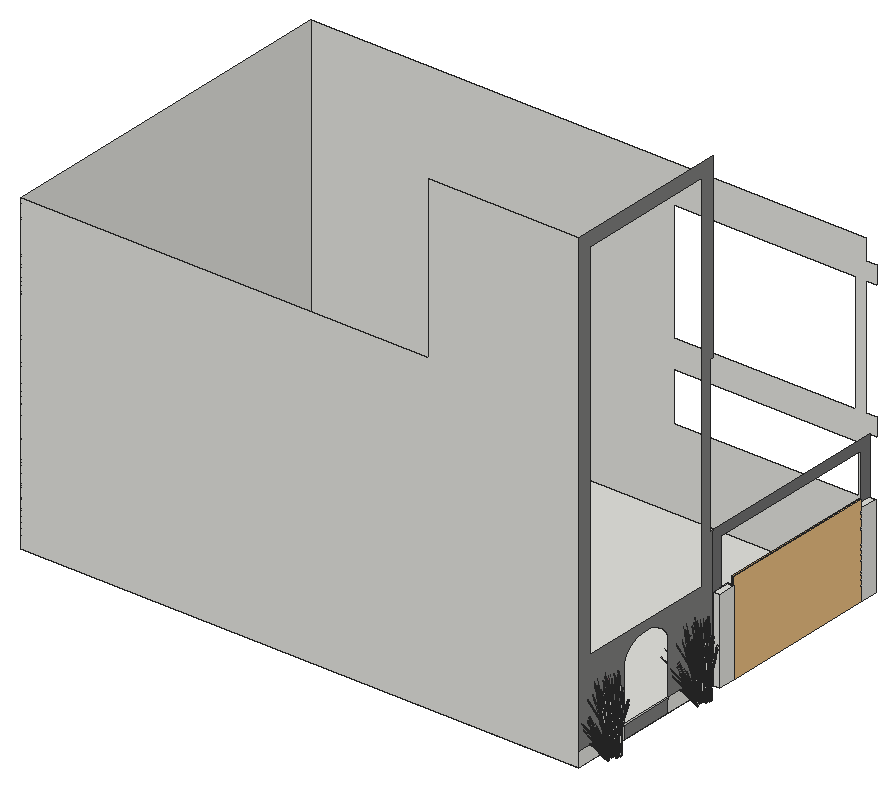
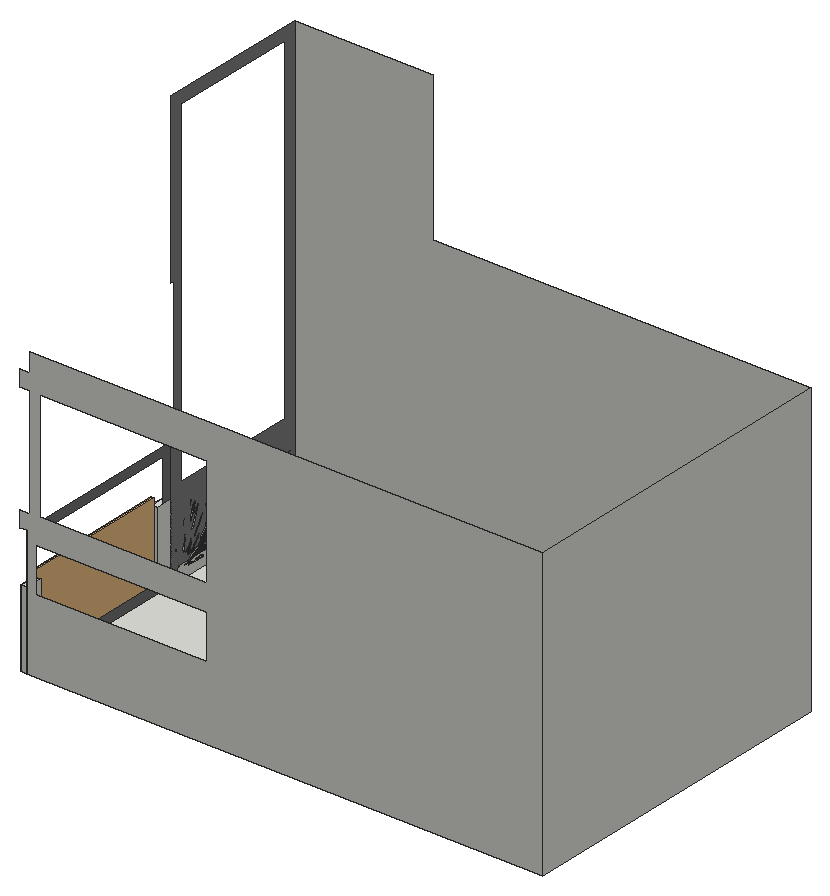
# SketchUp Ruby script. Lengths in inches.
U = 1.inch
M = Sketchup.active_model
def pt(a) = Geom::Point3d.new(a.map { |v| v * U })
def face(e, loops, mat)
  f = e.add_face(loops[0].map { |a| pt(a) })
  loops[1..].each { |l| e.add_face(l.map { |a| pt(a) }).erase! }
  f.material = f.back_material = mat if mat
  f
end
# faces: each face lists its corners as indices into pts; further lists are holes
def faces(e, pts, list, mat = nil) = list.each { |f| face(e, (f[0].is_a?(Array) ? f : [f]).map { |l| l.map { |i| pts[i] } }, mat) }
# xy, xz, yz: faces in a plane at the given z, y or x. An outline is a flat list of corners, or four numbers for a rectangle; further outlines are holes
def ring(l) = l.size == 4 ? [[l[0], l[1]], [l[2], l[1]], [l[2], l[3]], [l[0], l[3]]] : l.each_slice(2).to_a
def flat(e, list, mat, &to3) = list.each { |f| face(e, (f[0].is_a?(Array) ? f : [f]).map { |l| ring(l).map { |u, v| to3.(u, v) } }, mat) }
def xy(e, z, list, mat = nil) = flat(e, list, mat) { |x, y| [x, y, z] }
def xz(e, y, list, mat = nil) = flat(e, list, mat) { |x, z| [x, y, z] }
def yz(e, x, list, mat = nil) = flat(e, list, mat) { |y, z| [x, y, z] }
def lines(e, pts, list) = list.each { |a, b| e.add_line(pt(pts[a]), pt(pts[b])) }
# prism: a flat outline (further loops are holes) pulled along v
def prism(e, loops, v, mat = nil)
  f = face(e, loops, mat); d = Geom::Vector3d.new(v.map { |x| x * U })
  f.pushpull(f.normal.samedirection?(d) ? d.length : -d.length)
end
def box(e, o, s, mat = nil) = prism(e, [[o, [o[0] + s[0], o[1], o[2]], [o[0] + s[0], o[1] + s[1], o[2]], [o[0], o[1] + s[1], o[2]]]], [0, 0, s[2]], mat)
def at(x, y, z, deg = 0) = Geom::Transformation.translation(pt([x, y, z])) * Geom::Transformation.rotation(ORIGIN, Z_AXIS, deg.degrees)
def axes(o, x, y, z) = Geom::Transformation.new([*x, 0, *y, 0, *z, 0, *pt(o).to_a, 1])
def part(name) = M.definitions.add(name)
# library, detail: a bought-in or finely detailed component or shape, given as its bounding box
def library(name, o, s) = part(name).tap { |d| box(d.entities, o, s) }
def detail(e, o, s) = box(e.add_group.entities, o, s)
def put(e, d, t, mat = nil) = e.add_instance(d, t).tap { |i| i.material = mat if mat }
def group(e, t, mat = nil) = e.add_group.tap { |g| g.transformation = t; g.material = mat if mat }.entities
root = M.entities
M.materials.add("LightPink_Translucent").color = [144, 107, 117]
M.materials["LightPink_Translucent"].alpha = 0.75
M.materials.add("M05_Graphite_Haze").color = [114, 114, 114]
M.materials.add("ThomThom - Waistcoat2").color = [127, 127, 126]
c1 = part("blade")
p = [[2.15,0.21,22],[0,0.17,0],[0.09,0.45,0],[2.18,0.31,22],[2.29,0.31,22],[0.38,0.45,0],
  [2.48,0.24,33],[2.49,0.24,33],[2.48,0.22,33]]
faces(c1.entities,p,[[0,1,2,3],[4,5,2,3],[6,3,4,7],[8,0,3,6]])
c2 = part("seeds")
p = [[0.3,-0.1,1.38],[-0.01,-0.03,1.59],[-0.01,-0.03,0.03],[0.14,-0.07,-0.07],[0.29,-0.03,3],[0.15,0.01,3.11]]
faces(c2.entities,p,[[0,1,2,3],[1,0,4,5]],"LightPink_Translucent")
c3 = part("blade with seeds")
put(c3.entities,c1,at(0,0,0))
put(c3.entities,c2,axes([2.4,0.25,30.99],[1.5799,-0.05474,1.17369],[-0.12525,1.92788,0.29478],[-0.07173,-0.02425,1.56792]))
c4 = library("Modern+Gate+1",[0,0,0],[118.11,1.97,78.74])
box(root,[480,144,0],[6,15.46,72])
box(root,[480,295.78,0],[6,15.46,72])
xy(root,0,[[0,0,480,312]])
xz(root,0,[[0,0,480,0,480,408,351.33,408,351.33,270,0,270]])
xz(root,312,[[[0,0,0,270,477,270,477,252,486,252,486,237,312,237,312,135,468,135,468,237,477,237,477,135,486,135,486,120,480,120,480,0],[312,69,471,111]]])
yz(root,0,[[0,0,312,270]])
yz(root,480,[[0,0,48,0,48,11.26,96,11.26,96,12,0,12],[96,0,136.05,12]])
yz(root,480,[[[144,0,312,120],[153,9,303,111]]],"M05_Graphite_Haze")
yz(root,480,[[[136.05,0,144,0,144,120,141,120,141,252,144,252,144,408,0,408,0,12,48,12,48,60,50.74,64,54.14,67.47,58.1,70.28,62.48,72.35,67.17,73.62,72,74.05,76.83,73.62,81.52,72.35,85.9,70.28,89.86,67.47,93.26,64,96,60,96,12,136.05,12],[12,81.33,132,396]],[48,0,96,11.26]],"ThomThom - Waistcoat2")
put(root,c3,axes([486.59,117.58,3.875],[0.50831,-0.02346,1.71376],[-0.33721,1.01661,0.13857],[-0.72439,-0.06288,0.73262]))
put(root,c3,axes([486.59,21.58,3.875],[0.50831,-0.02346,1.71376],[-0.33721,1.01661,0.13857],[-0.72439,-0.06288,0.73262]))
put(root,c3,axes([486.8,119.375,3.875],[0.42521,-0.21906,1.71376],[0.35798,1.01226,0.13857],[-0.66754,0.22878,0.73262]))
put(root,c3,axes([486.8,23.375,3.875],[0.42521,-0.21906,1.71376],[0.35798,1.01226,0.13857],[-0.66754,0.22878,0.73262]))
put(root,c3,axes([485.48,121.1,2.59],[0.42589,0.08502,1.43002],[0.2745,0.86839,-0.30754],[-0.57851,0.16255,0.61141]))
put(root,c3,axes([485.48,25.1,2.59],[0.42589,0.08502,1.43002],[0.2745,0.86839,-0.30754],[-0.57851,0.16255,0.61141]))
put(root,c3,axes([489.25,118.32,3.34],[0.34834,-0.14982,1.77064],[0.12012,1.04605,0.13857],[-0.75452,0.1388,0.63284]))
put(root,c3,axes([489.25,22.32,3.34],[0.34834,-0.14982,1.77064],[0.12012,1.04605,0.13857],[-0.75452,0.1388,0.63284]))
put(root,c3,axes([488.11,116.64,4.98],[-1.22504,-0.02494,-0.71045],[0.08228,-1.05005,0.08574],[-0.51899,-0.11081,1.00501]))
put(root,c3,axes([488.11,20.64,4.98],[-1.22504,-0.02494,-0.71045],[0.08228,-1.05005,0.08574],[-0.51899,-0.11081,1.00501]))
put(root,c3,axes([487.125,116.9,2.59],[0.23927,0.28834,1.43002],[-0.55135,0.78376,-0.30754],[-0.56612,-0.18733,0.61141]))
put(root,c3,axes([487.125,20.9,2.59],[0.23927,0.28834,1.43002],[-0.55135,0.78376,-0.30754],[-0.56612,-0.18733,0.61141]))
put(root,c3,axes([486.14,118.46,4.53],[-1.01846,-0.28891,-0.35414],[0.29705,-0.84289,0.4572],[-0.41005,0.07729,0.87481]))
put(root,c3,axes([486.14,22.46,4.53],[-1.01846,-0.28891,-0.35414],[0.29705,-0.84289,0.4572],[-0.41005,0.07729,0.87481]))
put(root,c3,axes([487.55,115.95,3.875],[0.45521,0.17844,1.71376],[-0.94204,0.74856,0.13857],[-0.58713,-0.33769,0.73262]))
put(root,c3,axes([487.55,19.95,3.875],[0.45521,0.17844,1.71376],[-0.94204,0.74856,0.13857],[-0.58713,-0.33769,0.73262]))
put(root,c3,axes([486.84,118.89,4.68],[-0.332,0.94205,-0.51099],[-1.13828,-0.3229,-0.3958],[-0.45829,0.08638,0.97773]))
put(root,c3,axes([486.84,22.89,4.68],[-0.332,0.94205,-0.51099],[-1.13828,-0.3229,-0.3958],[-0.45829,0.08638,0.97773]))
put(root,c3,axes([487.7,116.85,4.68],[-0.88986,0.68603,-0.51099],[-0.77932,-0.72471,-0.3958],[-0.45212,-0.10438,0.97773]))
put(root,c3,axes([487.7,20.85,4.68],[-0.88986,0.68603,-0.51099],[-0.77932,-0.72471,-0.3958],[-0.45212,-0.10438,0.97773]))
put(root,c3,axes([486.27,118.83,1.49],[0.03108,0.16322,1.76342],[-0.62654,0.85237,-0.26939],[-0.44504,-0.04296,0.30037]))
put(root,c3,axes([486.27,22.83,1.49],[0.03108,0.16322,1.76342],[-0.62654,0.85237,-0.26939],[-0.44504,-0.04296,0.30037]))
put(root,c3,axes([484.59,122.92,2.77],[0.51072,-0.46938,1.1486],[0.20153,0.74307,0.84392],[-0.36908,0.13305,0.25299]))
put(root,c3,axes([484.59,26.92,2.77],[0.51072,-0.46938,1.1486],[0.20153,0.74307,0.84392],[-0.36908,0.13305,0.25299]))
put(root,c3,axes([487.375,116.21,4.53],[-0.69728,-0.64842,-0.35414],[0.79619,-0.61382,0.4572],[-0.40453,-0.09339,0.87481]))
put(root,c3,axes([487.375,20.21,4.53],[-0.69728,-0.64842,-0.35414],[0.79619,-0.61382,0.4572],[-0.40453,-0.09339,0.87481]))
put(root,c3,axes([488.36,120.06,3.875],[0.30609,-0.31822,1.71376],[0.77286,0.85893,0.13857],[-0.53009,0.39116,0.73262]))
put(root,c3,axes([488.36,24.06,3.875],[0.30609,-0.31822,1.71376],[0.77286,0.85893,0.13857],[-0.53009,0.39116,0.73262]))
put(root,c3,axes([486.52,120.89,4.53],[-1.06674,0.14801,-0.35414],[-0.28168,-0.84611,0.4572],[-0.30569,0.22726,0.87481]))
put(root,c3,axes([486.52,24.89,4.53],[-1.06674,0.14801,-0.35414],[-0.28168,-0.84611,0.4572],[-0.30569,0.22726,0.87481]))
put(root,c3,axes([485.93,123.4,1.49],[0.16438,0.10347,1.76342],[0.27873,0.95868,-0.26939],[-0.36432,0.20444,0.30037]))
put(root,c3,axes([485.93,27.4,1.49],[0.16438,0.10347,1.76342],[0.27873,0.95868,-0.26939],[-0.36432,0.20444,0.30037]))
put(root,c3,axes([485.7,117.76,2.77],[0.78239,-0.07411,1.1486],[-0.49629,0.65296,0.84392],[-0.38663,-0.09795,0.25299]))
put(root,c3,axes([485.7,21.76,2.77],[0.78239,-0.07411,1.1486],[-0.49629,0.65296,0.84392],[-0.38663,-0.09795,0.25299]))
put(root,c3,axes([488.13,120.84,3.875],[0.22818,-0.35597,1.71376],[0.95725,0.73667,0.13857],[-0.43183,0.45914,0.73262]))
put(root,c3,axes([488.13,24.84,3.875],[0.22818,-0.35597,1.71376],[0.95725,0.73667,0.13857],[-0.43183,0.45914,0.73262]))
put(root,c3,axes([487.4,120.99,4.68],[0.31482,0.94565,-0.51099],[-1.19224,0.16542,-0.3958],[-0.34166,0.254,0.97773]))
put(root,c3,axes([487.4,24.99,4.68],[0.31482,0.94565,-0.51099],[-1.19224,0.16542,-0.3958],[-0.34166,0.254,0.97773]))
put(root,c3,axes([490.37,120.31,2.06],[-1.27479,-0.1698,-0.62353],[0.26901,-1.04736,-0.16365],[-0.38043,-0.12691,1.37633]))
put(root,c3,axes([490.37,24.31,2.06],[-1.27479,-0.1698,-0.62353],[0.26901,-1.04736,-0.16365],[-0.38043,-0.12691,1.37633]))
put(root,c3,axes([490.24,115.4,4.98],[-1.04497,-0.50058,-0.71045],[0.74264,-0.8772,0.08574],[-0.3786,-0.29889,1.00501]))
put(root,c3,axes([490.24,19.4,4.98],[-1.04497,-0.50058,-0.71045],[0.74264,-0.8772,0.08574],[-0.3786,-0.29889,1.00501]))
put(root,c3,axes([489.75,115.43,4.68],[-1.20928,0.24619,-0.51099],[-0.21154,-0.93233,-0.3958],[-0.32481,-0.26718,0.97773]))
put(root,c3,axes([489.75,19.43,4.68],[-1.20928,0.24619,-0.51099],[-0.21154,-0.93233,-0.3958],[-0.32481,-0.26718,0.97773]))
put(root,c3,axes([488.7,122.29,2.02],[-1.14694,-0.51783,-0.49651],[0.68554,-0.92854,0],[-0.26122,-0.11794,1.57504]))
put(root,c3,axes([488.7,26.29,2.02],[-1.14694,-0.51783,-0.49651],[0.68554,-0.92854,0],[-0.26122,-0.11794,1.57504]))
put(root,c3,axes([488.19,114.58,1.49],[-0.11871,0.13643,1.76342],[-1.19964,0.29415,-0.26939],[-0.2898,-0.26759,0.30037]))
put(root,c3,axes([488.19,18.58,1.49],[-0.11871,0.13643,1.76342],[-1.19964,0.29415,-0.26939],[-0.2898,-0.26759,0.30037]))
put(root,c3,axes([489.39,122.92,2.375],[-0.7662,1.03778,0],[-1.28187,-0.57875,-0.51607],[-0.29196,-0.13181,1.63711]))
put(root,c3,axes([489.39,26.92,2.375],[-0.7662,1.03778,0],[-1.28187,-0.57875,-0.51607],[-0.29196,-0.13181,1.63711]))
put(root,c3,axes([488,124.42,2.59],[0.38672,-0.16338,1.43002],[0.95481,0.49262,-0.30754],[-0.28419,0.42626,0.61141]))
put(root,c3,axes([488,28.42,2.59],[0.38672,-0.16338,1.43002],[0.95481,0.49262,-0.30754],[-0.28419,0.42626,0.61141]))
put(root,c3,axes([487.45,115.1,2.13],[-0.35352,0.84566,-0.03893],[-1.08806,-0.26014,-0.17649],[-0.1652,-0.13832,0.58215]))
put(root,c3,axes([487.45,19.1,2.13],[-0.35352,0.84566,-0.03893],[-1.08806,-0.26014,-0.17649],[-0.1652,-0.13832,0.58215]))
put(root,c3,axes([489.07,114.04,2.59],[-0.07421,0.33879,1.43002],[-1.08488,0.28361,-0.30754],[-0.25359,-0.4379,0.61141]))
put(root,c3,axes([489.07,18.04,2.59],[-0.07421,0.33879,1.43002],[-1.08488,0.28361,-0.30754],[-0.25359,-0.4379,0.61141]))
put(root,c3,axes([489.43,114.92,3.875],[0.28013,0.33252,1.71376],[-1.29445,0.27994,0.13857],[-0.29256,-0.52202,0.73262]))
put(root,c3,axes([489.43,18.92,3.875],[0.28013,0.33252,1.71376],[-1.29445,0.27994,0.13857],[-0.29256,-0.52202,0.73262]))
put(root,c3,axes([491.8125,120.46,2.67],[-1.23732,0.68758,-0.29095],[-0.8228,-0.97154,-0.50002],[-0.30528,-0.09867,1.59708]))
put(root,c3,axes([491.8125,24.46,2.67],[-1.23732,0.68758,-0.29095],[-0.8228,-0.97154,-0.50002],[-0.30528,-0.09867,1.59708]))
put(root,c3,axes([489.88,114.74,4.53],[-0.18927,-0.83419,-0.35414],[1.08199,-0.22027,0.4572],[-0.29062,-0.23905,0.87481]))
put(root,c3,axes([489.88,18.74,4.53],[-0.18927,-0.83419,-0.35414],[1.08199,-0.22027,0.4572],[-0.29062,-0.23905,0.87481]))
put(root,c3,axes([486.86,118.96,2.375],[-1.53239,0,0],[0,-1.1575,-0.51607],[0,-0.26363,1.63711]))
put(root,c3,axes([486.86,22.96,2.375],[-1.53239,0,0],[0,-1.1575,-0.51607],[0,-0.26363,1.63711]))
put(root,c3,axes([489.01,121.9,2.03],[-0.28787,-0.90242,-0.30978],[1.14332,-0.25625,0.30978],[-0.23049,-0.10406,1.38974]))
put(root,c3,axes([489.01,25.9,2.03],[-0.28787,-0.90242,-0.30978],[1.14332,-0.25625,0.30978],[-0.23049,-0.10406,1.38974]))
put(root,c3,axes([488.39,122.85,4.53],[-0.82919,0.54528,-0.35414],[-0.78493,-0.62262,0.4572],[-0.11943,0.31634,0.87481]))
put(root,c3,axes([488.39,26.85,4.53],[-0.82919,0.54528,-0.35414],[-0.78493,-0.62262,0.4572],[-0.11943,0.31634,0.87481]))
put(root,c4,axes([486,159.46,0],[0,1.15423,0],[-1,0,0],[0,0,1]))
put(root,c3,axes([492.64,121.21,2.06],[-0.82544,0.77843,-0.62353],[-1.0254,-0.70586,-0.16365],[-0.33076,0.19418,1.37633]))
put(root,c3,axes([492.64,25.21,2.06],[-0.82544,0.77843,-0.62353],[-1.0254,-0.70586,-0.16365],[-0.33076,0.19418,1.37633]))
put(root,c3,axes([488.05,118.66,2.33],[-1.1399,0.87071,0.30756],[-1.1406,-0.86155,-0.36492],[-0.03981,-0.24727,1.64885]))
put(root,c3,axes([488.05,22.66,2.33],[-1.1399,0.87071,0.30756],[-1.1406,-0.86155,-0.36492],[-0.03981,-0.24727,1.64885]))
put(root,c3,axes([492.74,121.07,3.33],[1.05902,0.41762,1.51261],[-1.03748,0.89969,0.59816],[-0.46471,-0.53324,1.26806]))
put(root,c3,axes([492.74,25.07,3.33],[1.05902,0.41762,1.51261],[-1.03748,0.89969,0.59816],[-0.46471,-0.53324,1.26806]))
put(root,c3,axes([488.7,113.49,2.77],[0.63926,0.36046,1.1486],[-0.93099,0.21668,0.84392],[-0.1992,-0.27702,0.25299]))
put(root,c3,axes([488.7,17.49,2.77],[0.63926,0.36046,1.1486],[-0.93099,0.21668,0.84392],[-0.1992,-0.27702,0.25299]))
put(root,c3,axes([493.2,120.78,2.46],[-1.19666,-0.83357,-0.25192],[1.00694,-0.93603,0.5513],[-0.32224,0.09751,1.68216]))
put(root,c3,axes([493.2,24.78,2.46],[-1.19666,-0.83357,-0.25192],[1.00694,-0.93603,0.5513],[-0.32224,0.09751,1.68216]))
put(root,c3,axes([491.03,119.98,2.21],[-0.73619,-0.86927,-0.44739],[1.11511,-0.61213,0.21531],[-0.23824,-0.10756,1.43643]))
put(root,c3,axes([491.03,23.98,2.21],[-0.73619,-0.86927,-0.44739],[1.11511,-0.61213,0.21531],[-0.23824,-0.10756,1.43643]))
put(root,c3,axes([488.95,122.27,5.34],[-0.03189,0.95798,-0.7886],[-1.34277,-0.06434,0.09517],[-0.14171,0.40585,1.11556]))
put(root,c3,axes([488.95,26.27,5.34],[-0.03189,0.95798,-0.7886],[-1.34277,-0.06434,0.09517],[-0.14171,0.40585,1.11556]))
put(root,c3,axes([488.92,124.96,2.77],[-0.03171,-0.6158,1.1486],[0.7925,0.43922,0.84392],[-0.15586,0.29352,0.25299]))
put(root,c3,axes([488.92,28.96,2.77],[-0.03171,-0.6158,1.1486],[0.7925,0.43922,0.84392],[-0.15586,0.29352,0.25299]))
put(root,c3,axes([492.6,120.6,2.21],[-1.33077,0.06393,-0.44739],[-0.12035,-1.06125,0.21531],[-0.23824,0.10756,1.43643]))
put(root,c3,axes([492.6,24.6,2.21],[-1.33077,0.06393,-0.44739],[-0.12035,-1.06125,0.21531],[-0.23824,0.10756,1.43643]))
put(root,c3,axes([490.05,122.375,2.48],[1.14694,0.51783,0.49651],[-0.68554,0.92854,0],[-0.26122,-0.11794,1.57504]))
put(root,c3,axes([490.05,26.375,2.48],[1.14694,0.51783,0.49651],[-0.68554,0.92854,0],[-0.26122,-0.11794,1.57504]))
put(root,c3,axes([488.5,123.62,3.36],[0.02693,-0.53464,1.54345],[1.21102,0.2824,0.21329],[-0.10493,0.5698,0.72882]))
put(root,c3,axes([488.5,27.62,3.36],[0.02693,-0.53464,1.54345],[1.21102,0.2824,0.21329],[-0.10493,0.5698,0.72882]))
put(root,c3,axes([491.14,120.47,2.4375],[0.32481,-1.2272,-0.23429],[1.54007,0.21392,0.51271],[-0.26911,-0.16947,1.5644]))
put(root,c3,axes([491.14,24.47,2.4375],[0.32481,-1.2272,-0.23429],[1.54007,0.21392,0.51271],[-0.26911,-0.16947,1.5644]))
put(root,c3,axes([491.7,120.76,2.62],[-0.23642,0.92427,0.1448],[-1.15506,-0.16044,-0.41347],[-0.21021,-0.09491,1.26744]))
put(root,c3,axes([491.7,24.76,2.62],[-0.23642,0.92427,0.1448],[-1.15506,-0.16044,-0.41347],[-0.21021,-0.09491,1.26744]))
put(root,c3,axes([494,123.34,2.02],[-1.14694,0.51783,-0.49651],[-0.68554,-0.92854,0],[-0.26122,0.11794,1.57504]))
put(root,c3,axes([494,27.34,2.02],[-1.14694,0.51783,-0.49651],[-0.68554,-0.92854,0],[-0.26122,0.11794,1.57504]))
put(root,c3,axes([487.21,118.18,2.02],[0,-1.03566,-0.49651],[1.37109,0,0],[0,-0.23588,1.57504]))
put(root,c3,axes([487.21,22.18,2.02],[0,-1.03566,-0.49651],[1.37109,0,0],[0,-0.23588,1.57504]))
put(root,c3,axes([487.79,119.14,2.48],[0,1.03566,0.49651],[-1.37109,0,0],[0,-0.23588,1.57504]))
put(root,c3,axes([487.79,23.14,2.48],[0,1.03566,0.49651],[-1.37109,0,0],[0,-0.23588,1.57504]))
put(root,c3,axes([494.07,123.06,2.19],[-0.75665,-1.04141,-0.05142],[1.28187,-0.57875,0.51607],[-0.31588,0.09915,1.6363]))
put(root,c3,axes([494.07,27.06,2.19],[-0.75665,-1.04141,-0.05142],[1.28187,-0.57875,0.51607],[-0.31588,0.09915,1.6363]))
put(root,c3,axes([489.22,122.59,5],[0.87728,0.69587,-0.5672],[-0.92674,0.60943,-0.43934],[-0.13348,0.35356,1.08528]))
put(root,c3,axes([489.22,26.59,5],[0.87728,0.69587,-0.5672],[-0.92674,0.60943,-0.43934],[-0.13348,0.35356,1.08528]))
put(root,c3,axes([493.73,122.93,2.03],[-1.14332,-0.25625,-0.30978],[0.28787,-0.90242,0.30978],[-0.23049,0.10406,1.38974]))
put(root,c3,axes([493.73,26.93,2.03],[-1.14332,-0.25625,-0.30978],[0.28787,-0.90242,0.30978],[-0.23049,0.10406,1.38974]))
put(root,c3,axes([490.79,119.375,2.67],[-1.38012,-0.49416,-0.29095],[0.66454,-1.04299,-0.50002],[-0.04337,-0.25608,1.59708]))
put(root,c3,axes([490.79,23.375,2.67],[-1.38012,-0.49416,-0.29095],[0.66454,-1.04299,-0.50002],[-0.04337,-0.25608,1.59708]))
put(root,c3,axes([494.38,119.07,2.84],[-0.03348,-0.97511,1.41272],[1.51511,0.25277,0.59816],[-0.35835,0.53357,1.3335]))
put(root,c3,axes([494.38,23.07,2.84],[-0.03348,-0.97511,1.41272],[1.51511,0.25277,0.59816],[-0.35835,0.53357,1.3335]))
put(root,c3,axes([488.27,123.63,2.82],[1.11329,-0.1834,0.06507],[0.25594,0.73887,-0.86304],[-0.07058,0.37403,0.7736]))
put(root,c3,axes([488.27,27.63,2.82],[1.11329,-0.1834,0.06507],[0.25594,0.73887,-0.86304],[-0.07058,0.37403,0.7736]))
put(root,c3,axes([493.53,120.3125,2.67],[0.1428,1.18174,-0.29095],[-1.48733,0.07145,-0.50002],[-0.26191,0.15741,1.59708]))
put(root,c3,axes([493.53,24.3125,2.67],[0.1428,1.18174,-0.29095],[-1.48733,0.07145,-0.50002],[-0.26191,0.15741,1.59708]))
put(root,c3,axes([490.17,118.33,2.1],[-0.50328,-1.06202,-0.69835],[1.44974,-0.38248,-0.18329],[-0.05563,-0.35963,1.54149]))
put(root,c3,axes([490.17,22.33,2.1],[-0.50328,-1.06202,-0.69835],[1.44974,-0.38248,-0.18329],[-0.05563,-0.35963,1.54149]))
put(root,c3,axes([492.4375,114.99,4.68],[-1.20468,-0.25962,-0.51099],[0.41292,-0.89013,-0.3958],[-0.11046,-0.35838,0.97773]))
put(root,c3,axes([492.4375,18.99,4.68],[-1.20468,-0.25962,-0.51099],[0.41292,-0.89013,-0.3958],[-0.11046,-0.35838,0.97773]))
put(root,c3,axes([490.22,121.59,3.875],[-0.02999,-0.3975,1.71376],[1.30002,0.26369,0.13857],[-0.08041,0.56647,0.73262]))
put(root,c3,axes([490.22,25.59,3.875],[-0.02999,-0.3975,1.71376],[1.30002,0.26369,0.13857],[-0.08041,0.56647,0.73262]))
put(root,c3,axes([487.79,118.2,2.03],[0.85545,-0.64616,-0.30978],[0.85545,0.64616,0.30978],[0,-0.20813,1.38974]))
put(root,c3,axes([487.79,22.2,2.03],[0.85545,-0.64616,-0.30978],[0.85545,0.64616,0.30978],[0,-0.20813,1.38974]))
put(root,c3,axes([491.66,114.02,2.13],[-0.84686,0.59414,-0.03893],[-0.77596,-0.65071,-0.17649],[-0.05463,-0.18438,0.58215]))
put(root,c3,axes([491.66,18.02,2.13],[-0.84686,0.59414,-0.03893],[-0.77596,-0.65071,-0.17649],[-0.05463,-0.18438,0.58215]))
put(root,c3,axes([491.32,119.88,2.36],[1.54892,0.2182,0.45755],[-0.31522,1.23236,0.17955],[-0.22636,-0.119,1.58856]))
put(root,c3,axes([491.32,23.88,2.36],[1.54892,0.2182,0.45755],[-0.31522,1.23236,0.17955],[-0.22636,-0.119,1.58856]))
put(root,c3,axes([490.91,119.66,2.72],[-0.59459,0.93321,0.44739],[-1.23546,-0.44912,-0.21531],[0,-0.21512,1.43643]))
put(root,c3,axes([490.91,23.66,2.72],[-0.59459,0.93321,0.44739],[-1.23546,-0.44912,-0.21531],[0,-0.21512,1.43643]))
put(root,c3,axes([492.875,115.16,4.98],[-0.5849,-0.8421,-0.71045],[1.20401,-0.4693,0.08574],[-0.13677,-0.40688,1.00501]))
put(root,c3,axes([492.875,19.16,4.98],[-0.5849,-0.8421,-0.71045],[1.20401,-0.4693,0.08574],[-0.13677,-0.40688,1.00501]))
put(root,c3,axes([490.48,121.85,2.47],[1.31687,-0.27488,0.17642],[0.32517,1.02297,0.35086],[-0.11745,-0.14905,1.60407]))
put(root,c3,axes([490.48,25.85,2.47],[1.31687,-0.27488,0.17642],[0.32517,1.02297,0.35086],[-0.11745,-0.14905,1.60407]))
put(root,c3,axes([492.18,122.01,2.2],[-1.23546,-0.46496,0],[0.59459,-0.96613,0],[0,0,1.62707]))
put(root,c3,axes([492.18,26.01,2.2],[-1.23546,-0.46496,0],[0.59459,-0.96613,0],[0,0,1.62707]))
put(root,c3,axes([495.04,123.18,2.375],[0.7662,1.03778,0],[-1.28187,0.57875,-0.51607],[-0.29196,0.13181,1.63711]))
put(root,c3,axes([495.04,27.18,2.375],[0.7662,1.03778,0],[-1.28187,0.57875,-0.51607],[-0.29196,0.13181,1.63711]))
put(root,c3,axes([494.4,121.91,2.47],[0.35402,-1.02926,0.17642],[1.29548,0.29127,0.35086],[-0.22379,0.00501,1.60407]))
put(root,c3,axes([494.4,25.91,2.47],[0.35402,-1.02926,0.17642],[1.29548,0.29127,0.35086],[-0.22379,0.00501,1.60407]))
put(root,c3,axes([493.8,120.54,2.62],[0.90538,0.62224,0.1448],[-0.75521,0.70202,-0.41347],[-0.21021,0.09491,1.26744]))
put(root,c3,axes([493.8,24.54,2.62],[0.90538,0.62224,0.1448],[-0.75521,0.70202,-0.41347],[-0.21021,0.09491,1.26744]))
put(root,c3,axes([493.48,119.77,2.3],[-1.1399,-0.8914,-0.06131],[1.1406,-0.89194,0],[-0.03981,-0.03113,1.75571]))
put(root,c3,axes([493.48,23.77,2.3],[-1.1399,-0.8914,-0.06131],[1.1406,-0.89194,0],[-0.03981,-0.03113,1.75571]))
put(root,c3,axes([493.78,120.09,2.72],[1.33077,-0.06393,0.44739],[0.12035,1.06125,-0.21531],[-0.23824,0.10756,1.43643]))
put(root,c3,axes([493.78,24.09,2.72],[1.33077,-0.06393,0.44739],[0.12035,1.06125,-0.21531],[-0.23824,0.10756,1.43643]))
put(root,c3,axes([494.11,122.53,2.33],[1.53422,0.33662,0.30756],[-0.38383,1.20322,-0.36492],[-0.25393,0.15059,1.64885]))
put(root,c3,axes([494.11,26.53,2.33],[1.53422,0.33662,0.30756],[-0.38383,1.20322,-0.36492],[-0.25393,0.15059,1.64885]))
put(root,c3,axes([491.87,113.3,1.49],[-0.20555,0.03731,1.76342],[-1.13672,-0.42002,-0.26939],[0.01907,-0.35034,0.30037]))
put(root,c3,axes([491.87,17.3,1.49],[-0.20555,0.03731,1.76342],[-1.13672,-0.42002,-0.26939],[0.01907,-0.35034,0.30037]))
put(root,c3,axes([494.77,122.46,2.48],[1.14694,-0.51783,0.49651],[0.68554,0.92854,0],[-0.26122,0.11794,1.57504]))
put(root,c3,axes([494.77,26.46,2.48],[1.14694,-0.51783,0.49651],[0.68554,0.92854,0],[-0.26122,0.11794,1.57504]))
put(root,c3,axes([492.99,114.45,4.53],[0.36946,-0.79643,-0.35414],[1.07787,0.23229,0.4572],[-0.09883,-0.32066,0.87481]))
put(root,c3,axes([492.99,18.45,4.53],[0.36946,-0.79643,-0.35414],[1.07787,0.23229,0.4572],[-0.09883,-0.32066,0.87481]))
put(root,c3,axes([491.18,118.75,2.36],[0.53281,1.15808,0.45755],[-1.52239,0.4027,0.17955],[0.01861,-0.2128,1.58856]))
